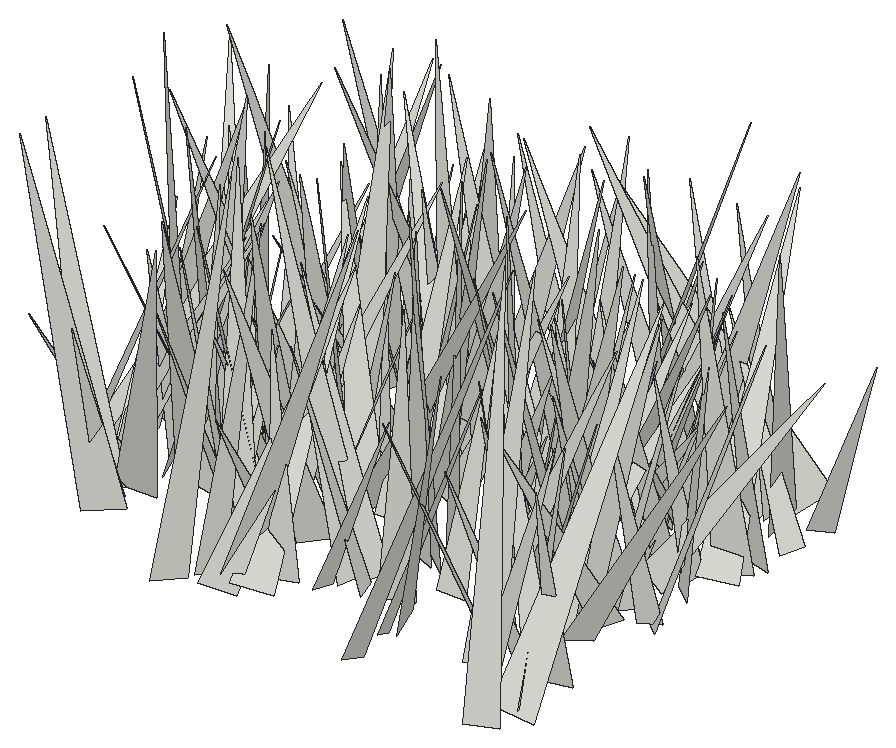
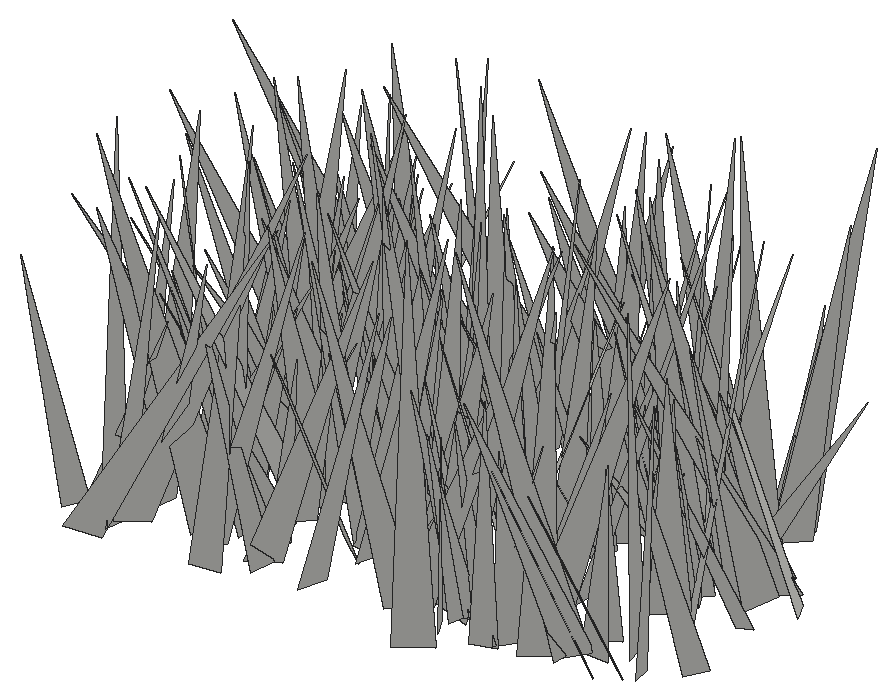
# SketchUp Ruby script. Lengths in inches.
U = 1.inch
M = Sketchup.active_model
def pt(a) = Geom::Point3d.new(a.map { |v| v * U })
def face(e, loops, mat)
  f = e.add_face(loops[0].map { |a| pt(a) })
  loops[1..].each { |l| e.add_face(l.map { |a| pt(a) }).erase! }
  f.material = f.back_material = mat if mat
  f
end
# faces: each face lists its corners as indices into pts; further lists are holes
def faces(e, pts, list, mat = nil) = list.each { |f| face(e, (f[0].is_a?(Array) ? f : [f]).map { |l| l.map { |i| pts[i] } }, mat) }
# xy, xz, yz: faces in a plane at the given z, y or x. An outline is a flat list of corners, or four numbers for a rectangle; further outlines are holes
def ring(l) = l.size == 4 ? [[l[0], l[1]], [l[2], l[1]], [l[2], l[3]], [l[0], l[3]]] : l.each_slice(2).to_a
def flat(e, list, mat, &to3) = list.each { |f| face(e, (f[0].is_a?(Array) ? f : [f]).map { |l| ring(l).map { |u, v| to3.(u, v) } }, mat) }
def xy(e, z, list, mat = nil) = flat(e, list, mat) { |x, y| [x, y, z] }
def xz(e, y, list, mat = nil) = flat(e, list, mat) { |x, z| [x, y, z] }
def yz(e, x, list, mat = nil) = flat(e, list, mat) { |y, z| [x, y, z] }
def lines(e, pts, list) = list.each { |a, b| e.add_line(pt(pts[a]), pt(pts[b])) }
# prism: a flat outline (further loops are holes) pulled along v
def prism(e, loops, v, mat = nil)
  f = face(e, loops, mat); d = Geom::Vector3d.new(v.map { |x| x * U })
  f.pushpull(f.normal.samedirection?(d) ? d.length : -d.length)
end
def box(e, o, s, mat = nil) = prism(e, [[o, [o[0] + s[0], o[1], o[2]], [o[0] + s[0], o[1] + s[1], o[2]], [o[0], o[1] + s[1], o[2]]]], [0, 0, s[2]], mat)
def at(x, y, z, deg = 0) = Geom::Transformation.translation(pt([x, y, z])) * Geom::Transformation.rotation(ORIGIN, Z_AXIS, deg.degrees)
def axes(o, x, y, z) = Geom::Transformation.new([*x, 0, *y, 0, *z, 0, *pt(o).to_a, 1])
def part(name) = M.definitions.add(name)
# library, detail: a bought-in or finely detailed component or shape, given as its bounding box
def library(name, o, s) = part(name).tap { |d| box(d.entities, o, s) }
def detail(e, o, s) = box(e.add_group.entities, o, s)
def put(e, d, t, mat = nil) = e.add_instance(d, t).tap { |i| i.material = mat if mat }
def group(e, t, mat = nil) = e.add_group.tap { |g| g.transformation = t; g.material = mat if mat }.entities
root = M.entities
c1 = part("fur_instance\#9")
p = [[0.8125,0,1.79],[0.67,-0.02,1.48],[0,-0.11,0],[0,0.11,0]]
faces(c1.entities,p,[[0,1,2,3]])
put(root,c1,axes([156.88,270.8125,-27.1],[4.55494,-1.38322,1.77977],[-1.90749,-4.50337,1.38185],[-1.20098,1.9065,4.55536]))
put(root,c1,axes([138.06,273.06,-27.1],[2.50523,-6.92108,2.84903],[-7.08461,-3.16179,-1.45116],[-2.41383,2.09672,7.21607]))
put(root,c1,axes([158.23,269.17,-27.1],[0.30584,8.28043,0.48557],[7.987,-0.4251,2.21855],[-2.2381,-0.38549,7.98355]))
put(root,c1,axes([151.5,273.3,-27.1],[6.22131,1.299,1.34326],[1.60809,-6.10017,-1.54868],[-0.95174,-1.81575,6.1639]))
put(root,c1,axes([158.52,273.24,-27.1],[1.07632,-4.38935,0.89904],[-4.4763,-1.09335,0.02097],[-0.19334,0.87825,4.51934]))
put(root,c1,axes([143.01,270.55,-27.1],[-6.71814,2.72987,2.53139],[2.23652,7.13443,-1.75826],[2.97626,0.8008,7.03521]))
put(root,c1,axes([155.51,273.35,-27.1],[-3.79986,-3.34827,0.10157],[-3.34083,3.7767,-0.4853],[-0.24505,0.43103,5.04126]))
put(root,c1,axes([137.81,273.82,-27.1],[2.72704,-3.27265,0.76108],[-3.17295,-2.83078,-0.80329],[-1.10537,0.05182,4.1835]))
put(root,c1,axes([138.07,274.83,-27.1],[2.36593,-6.95857,0.28973],[-6.83072,-2.25873,1.53056],[1.359,0.76137,7.18865]))
put(root,c1,axes([156.9,273.36,-27.1],[-0.5806,-4.0301,0.94816],[-3.96701,0.26756,-1.29192],[-1.18471,1.07913,3.86131]))
put(root,c1,axes([158.72,271.08,-27.1],[-4.5247,0.14497,1.56827],[-0.47946,4.4174,-1.79167],[1.5002,1.84904,4.15738]))
put(root,c1,axes([146.21,273.05,-27.1],[-1.45922,4.42701,2.15741],[4.90506,1.50733,0.22462],[0.43952,-2.12407,4.65589]))
put(root,c1,axes([144.89,271.98,-27.1],[7.47756,-1.51643,1.55812],[-1.8154,-7.42558,1.48539],[-1.19651,1.78955,7.48379]))
put(root,c1,axes([144.78,271.08,-27.1],[-3.66435,5.27166,1.90181],[4.6134,4.12758,-2.55233],[3.18179,0.08644,5.89097]))
put(root,c1,axes([151.63,270.18,-27.1],[7.3603,1.92647,1.4977],[1.22652,-7.03518,3.02165],[-2.10951,2.63124,6.98247]))
put(root,c1,axes([144.33,275.14,-27.1],[1.81992,-3.21241,0.00061],[-3.09433,-1.75321,-0.99152],[-0.86298,-0.48823,3.55649]))
put(root,c1,axes([143.84,271.83,-27.1],[-6.0255,1.4926,2.28597],[0.94971,6.33899,-1.63567],[2.5596,1.16168,5.98825]))
put(root,c1,axes([147.59,273.53,-27.1],[4.04534,-0.8517,0.30361],[-0.87788,-4.03293,0.38361],[-0.21657,0.43867,4.11619]))
put(root,c1,axes([158.59,270.49,-27.1],[-1.16046,8.00046,0.20395],[7.87345,1.17823,-1.41992],[1.43448,0.00519,7.95851]))
put(root,c1,axes([148.91,274.3125,-27.1],[-4.66141,-1.64687,0.68606],[-1.65466,4.70851,0.06011],[0.66704,0.1713,4.94341]))
put(root,c1,axes([145.32,276.02,-27.1],[2.99002,-5.93259,1.12286],[-5.76165,-3.17812,-1.449],[-1.8055,0.31717,6.48354]))
put(root,c1,axes([141.33,276.06,-27.1],[-4.0085,-3.44331,0.94309],[-3.06456,4.04605,1.74695],[1.83147,-0.76613,4.98725]))
put(root,c1,axes([150.23,274.4,-27.1],[2.8988,-5.16102,2.16058],[-5.5292,-3.01461,0.21733],[-0.85564,1.9958,5.91539]))
put(root,c1,axes([144.27,273.01,-27.1],[-5.43034,-1.89464,0.64767],[-1.9986,5.01546,-2.08529],[-0.12137,2.18018,5.36002]))
put(root,c1,axes([137.33,274.07,-27.1],[-5.93712,3.87569,1.72238],[4.1151,5.9813,0.72589],[1.02637,-1.56207,7.0529]))
put(root,c1,axes([151.37,272.24,-27.1],[4.47299,1.54799,0.88013],[1.09405,-4.26651,1.94385],[-1.40498,1.60599,4.31572]))
put(root,c1,axes([138.91,277.35,-27.1],[6.44625,-4.17663,0.34492],[-3.99481,-6.31514,-1.81045],[-1.26676,-1.33867,7.46462]))
put(root,c1,axes([137.73,275.46,-27.1],[-0.38653,-3.78857,0.47263],[-3.40937,0.1287,-1.7566],[-1.71837,0.59684,3.37891]))
put(root,c1,axes([155.375,272.83,-27.1],[-6.19625,3.45387,1.64148],[3.0912,6.3638,-1.72156],[2.25127,0.76815,6.88178]))
put(root,c1,axes([155.24,274.8125,-27.1],[-4.18009,-2.38384,1.39005],[-2.61185,4.23208,-0.59649],[0.8906,1.22265,4.77494]))
put(root,c1,axes([143.08,274.33,-27.1],[-2.11891,6.73628,2.3501],[7.12334,2.13432,0.30482],[0.39806,-2.33612,7.05509]))
put(root,c1,axes([143.9,275.12,-27.1],[-3.99562,-4.42007,1.47298],[-4.65768,3.83659,-1.12173],[0.11293,1.84803,5.85182]))
put(root,c1,axes([142.59,274.4,-27.1],[-0.05946,3.80591,1.08242],[3.88392,0.26301,-0.71143],[0.75616,-1.05166,3.7393]))
put(root,c1,axes([145.18,273.13,-27.1],[5.43487,-1.88004,3.06705],[-2.9758,-5.47185,1.91904],[-2.02138,3.00059,5.42123]))
put(root,c1,axes([148.13,274.78,-27.1],[-8.02945,1.44749,0.94959],[1.4539,8.08421,-0.0293],[0.93976,-0.13944,8.15883]))
put(root,c1,axes([154.01,276.96,-27.1],[0.47232,-5.02453,0.37853],[-5.03579,-0.45765,0.20889],[0.17316,0.39615,5.04235]))
put(root,c1,axes([156.79,274.1875,-27.1],[-1.63602,4.97918,0.62205],[4.87533,1.42244,1.43652],[-1.18757,-1.0199,5.04036]))
put(root,c1,axes([157.19,277.71,-27.1],[2.87484,-4.36178,0.57915],[-3.91954,-2.85297,-2.03053],[-1.99945,-0.67874,4.81319]))
put(root,c1,axes([145.75,271.82,-27.1],[-4.59589,5.78444,0.11594],[5.4804,4.40003,-2.28044],[1.8543,1.33244,7.02721]))
put(root,c1,axes([143.55,276.78,-27.1],[-0.33962,-4.53633,0.58104],[-4.49375,0.22275,-0.88758],[-0.84975,0.63509,4.46159]))
put(root,c1,axes([142.36,278.12,-27.1],[6.58115,-3.41587,1.26301],[-3.10443,-6.62563,-1.74311],[-1.90417,-1.00387,7.20703]))
put(root,c1,axes([148.61,275.26,-27.1],[-5.80532,1.01557,0.17125],[1.00882,5.80466,-0.22508],[0.20737,0.19232,5.88918]))
put(root,c1,axes([138.62,278.8125,-27.1],[-3.25593,-5.45811,0.05054],[-5.36708,3.21208,1.12765],[0.99394,-0.53501,6.25464]))
put(root,c1,axes([149.46,277.47,-27.1],[-3.95013,-6.45103,2.53754],[-6.55598,4.42551,1.04517],[2.25256,1.56763,7.49179]))
put(root,c1,axes([153.51,275.75,-27.1],[2.52048,5.79703,1.2985],[5.75928,-2.03853,-2.07834],[1.45681,-1.97061,5.96983]))
put(root,c1,axes([135.79,275.93,-27.1],[4.10268,4.53992,0.30052],[4.35228,-3.79801,-2.04106],[1.3262,-1.58032,5.76861]))
put(root,c1,axes([142.4,276.375,-27.1],[-2.65775,-2.55388,1.91088],[-2.80676,3.05414,0.17806],[1.51521,1.17784,3.68161]))
put(root,c1,axes([148.78,277.39,-27.1],[-1.6159,-6.90986,2.38073],[-7.13771,2.01606,1.00679],[1.57067,2.05292,7.0245]))
put(root,c1,axes([137.93,277.77,-27.1],[3.7662,-3.06911,1.25827],[-2.92554,-3.97067,-0.92842],[-1.56328,0.03677,4.76883]))
put(root,c1,axes([151.5,275.9,-27.1],[-0.63443,5.02312,1.44392],[5.17666,0.80438,-0.52377],[0.72032,-1.3566,5.03586]))
put(root,c1,axes([157.02,276.14,-27.1],[5.8068,-2.41673,0.19711],[-2.36119,-5.5195,1.88633],[0.55156,1.81463,6.0001]))
put(root,c1,axes([136.15,276.54,-27.1],[3.52755,5.08967,0.59914],[4.90233,-3.13928,-2.19532],[1.49362,-1.71683,5.79042]))
put(root,c1,axes([139.86,276.4,-27.1],[1.56528,5.39191,1.82425],[5.61252,-1.77733,0.43748],[-0.9488,-1.61836,5.59744]))
put(root,c1,axes([155.9,277.65,-27.1],[-2.90009,-5.61636,1.60668],[-5.82709,2.65472,-1.23809],[-0.41218,1.98605,6.19848]))
put(root,c1,axes([153.88,278.1875,-27.1],[4.89387,1.35478,0.49174],[1.44124,-4.60961,-1.64362],[-0.00784,-1.71558,4.80457]))
put(root,c1,axes([146.14,277.15,-27.1],[3.85266,4.81198,3.39076],[5.17881,-4.69725,0.78179],[-2.79863,-2.06788,6.11449]))
put(root,c1,axes([155.28,279.84,-27.1],[3.26606,-6.16963,0.62937],[-6.14796,-3.31446,-0.58694],[-0.81426,0.27855,6.95607]))
put(root,c1,axes([138.24,279.3,-27.1],[-6.05203,-3.65216,2.90127],[-3.20675,6.70926,1.75646],[3.38709,-0.1736,6.84691]))
put(root,c1,axes([142.83,279.54,-27.1],[-3.8372,-2.33717,0.79383],[-2.01321,3.81242,1.493],[1.42812,-0.90538,4.23762]))
put(root,c1,axes([153.32,277.49,-27.1],[-6.66859,-2.01923,2.71074],[-2.32845,7.09045,-0.44648],[2.45024,1.24248,6.95328]))
put(root,c1,axes([158.25,278.68,-27.1],[1.30026,-4.12004,1.09762],[-4.18224,-1.45572,-0.50983],[-0.82967,0.8811,4.29016]))
put(root,c1,axes([136.82,275.79,-27.1],[-2.17484,4.53028,0.06229],[4.50087,2.16823,-0.54601],[0.51907,0.1805,4.99552]))
put(root,c1,axes([133.94,277.78,-27.1],[5.98281,3.47845,0.55141],[3.51313,-5.81778,-1.41742],[0.2481,-1.50052,6.77381]))
put(root,c1,axes([137.92,276.9,-27.1],[6.78168,2.91502,1.19431],[2.8839,-6.88568,0.43057],[-1.26762,-0.07012,7.36906]))
put(root,c1,axes([155.07,279.76,-27.1],[1.17594,-4.92519,0.34785],[-4.93492,-1.18388,-0.07952],[-0.1583,0.31979,5.06301]))
put(root,c1,axes([139.65,277.89,-27.1],[3.10895,3.01642,1.49943],[3.22004,-3.26039,-0.11754],[-0.98914,-1.13301,4.33019]))
put(root,c1,axes([151.19,278.72,-27.1],[2.68666,-2.71893,0.01615],[-2.65256,-2.616,0.85524],[0.59729,0.61233,3.72549]))
put(root,c1,axes([153.03,278.02,-27.1],[3.30994,1.56111,0.94089],[1.62723,-3.40964,-0.0672],[-0.82125,-0.46405,3.659]))
put(root,c1,axes([140.05,277.67,-27.1],[3.54809,3.00738,1.07129],[3.07779,-3.64774,0.04651],[-0.84804,-0.65624,4.65093]))
put(root,c1,axes([142.13,278.7,-27.1],[2.86459,-3.18276,1.27512],[-3.34476,-2.95943,0.1272],[-0.754,1.03614,4.28015]))
put(root,c1,axes([153.55,278.46,-27.1],[-3.32572,-4.76152,1.64129],[-5.0351,3.09772,-1.21581],[-0.11678,2.03921,5.67929]))
put(root,c1,axes([141.63,276.95,-27.1],[-0.67642,4.08917,0.12939],[3.98053,0.62749,0.97839],[-0.94522,-0.2838,4.0276]))
put(root,c1,axes([137.56,278.46,-27.1],[3.65064,-1.60023,0.53489],[-1.66152,-3.63138,0.47591],[-0.29361,0.65299,3.95745]))
put(root,c1,axes([142.9,277.91,-27.1],[0.16923,4.07191,1.2027],[4.12697,0.12503,-1.00402],[0.99752,-1.2081,3.94982]))
put(root,c1,axes([155.28,278.67,-27.1],[0.56131,-6.10589,2.64479],[-6.41112,0.21442,1.85565],[1.78167,2.69518,5.8441]))
put(root,c1,axes([138.05,277.61,-27.1],[3.6249,6.4726,3.15784],[6.5149,-4.45394,1.65071],[-3.06961,-1.8095,7.23254]))
put(root,c1,axes([156,276.26,-27.1],[0.77683,6.56918,0.32302],[6.56801,-0.79193,0.30978],[-0.34589,-0.28401,6.60769]))
put(root,c1,axes([157.04,278.98,-27.1],[-1.11932,5.12608,2.18052],[5.30702,0.30525,2.00664],[-1.6932,-2.43194,4.84799]))
put(root,c1,axes([135.375,278.34,-27.1],[6.77248,-2.83159,1.61361],[-3.13932,-6.6674,1.47599],[-0.87537,2.00399,7.19067]))
put(root,c1,axes([137.61,279.39,-27.1],[5.01911,-5.50348,2.14134],[-5.83765,-5.04831,0.7082],[-0.89193,2.07156,7.41473]))
put(root,c1,axes([140.43,281.86,-27.1],[-7.65526,-2.65251,1.50577],[-2.23878,7.64939,2.09305],[2.07148,-1.53532,7.82675]))
put(root,c1,axes([136.4,280.93,-27.1],[-5.36571,-5.00333,1.81378],[-4.95811,5.63559,0.87824],[1.93398,0.5664,7.28374]))
put(root,c1,axes([145.28,278.87,-27.1],[7.55011,-1.58138,0.22082],[-1.59514,-7.42262,1.38345],[0.0711,1.39915,7.58887]))
put(root,c1,axes([135.15,277.13,-27.1],[0.81957,8.13408,0.73803],[7.68253,-0.51597,-2.84467],[2.77248,-0.97476,7.66439]))
put(root,c1,axes([152.63,280.28,-27.1],[7.05562,-2.47543,1.6862],[-2.53392,-7.23407,-0.01726],[-1.59697,0.54154,7.47725]))
put(root,c1,axes([152.8,280.89,-27.1],[2.44609,-6.94499,1.47158],[-6.99231,-2.08787,1.76924],[1.22722,1.94671,7.14745]))
put(root,c1,axes([152.75,277.01,-27.1],[1.27817,7.72916,0.81529],[7.27012,-1.48113,2.64386],[-2.74773,-0.32349,7.37453]))
put(root,c1,axes([149.71,278.17,-27.1],[-6.21182,-1.68937,2.27799],[-2.42044,6.01654,-2.13837],[1.47806,2.75267,6.07191]))
put(root,c1,axes([135.25,279.7,-27.1],[2.3418,4.95634,1.60959],[5.19702,-2.35112,-0.32146],[-0.38351,-1.59595,5.4723]))
put(root,c1,axes([141.39,282.09,-27.1],[5.68928,-3.36377,1.44998],[-3.11585,-5.85243,-1.35122],[-1.92583,-0.46842,6.46971]))
put(root,c1,axes([147.45,278.09,-27.1],[5.41894,2.39891,1.8987],[1.67708,-5.5593,2.23748],[-2.55876,1.4367,5.48756]))
put(root,c1,axes([154.06,278.99,-27.1],[2.83544,5.2975,1.05869],[5.3487,-2.92083,0.29014],[-0.75876,-0.79328,6.00159]))
put(root,c1,axes([138.41,278.5,-27.1],[3.83996,1.68055,0.1423],[1.49178,-3.54944,1.66307],[-0.78682,1.47206,3.84756]))
put(root,c1,axes([146.5625,278.84,-27.1],[-1.26821,6.79621,1.34265],[6.86908,1.41065,-0.65215],[0.89826,-1.19212,6.8827]))
put(root,c1,axes([156.75,278.38,-27.1],[2.63197,4.07891,0.20518],[3.86496,-2.5665,1.44292],[-1.31973,0.61842,4.63495]))
put(root,c1,axes([138.45,279.76,-27.1],[-1.05429,4.67357,0.99792],[4.75005,0.91265,0.74413],[-0.52453,-1.12891,4.73287]))
put(root,c1,axes([137.33,279.15,-27.1],[3.31155,2.43431,1.59522],[1.82743,-3.61986,1.73033],[-2.2652,0.63849,3.72802]))
put(root,c1,axes([134.72,279.9375,-27.1],[1.36791,4.73736,0.76135],[4.55305,-1.0318,-1.76027],[1.51392,-1.17738,4.60599]))
put(root,c1,axes([152.19,280.03,-27.1],[3.72107,-3.56028,1.90501],[-4.03778,-3.30047,1.71878],[-0.03061,2.5656,4.85467]))
put(root,c1,axes([153.92,280.49,-27.1],[-4.56501,-1.69942,1.47091],[-1.97129,4.62695,-0.77219],[1.07964,1.26263,4.80947]))
put(root,c1,axes([149.29,281.62,-27.1],[1.54528,-3.8993,0.59524],[-3.77652,-1.27799,1.43226],[1.13873,1.05307,3.94222]))
put(root,c1,axes([158.62,278.38,-27.1],[3.88995,3.95886,0.07672],[3.75671,-3.72392,1.68217],[-1.25122,1.12695,5.2891]))
put(root,c1,axes([146.85,281.06,-27.1],[7.17764,0.6661,2.04171],[0.73913,-7.45363,-0.1667],[-2.01642,-0.36113,7.20655]))
put(root,c1,axes([147.49,280.95,-27.1],[1.43912,5.66343,2.07225],[5.60003,-0.46439,-2.61988],[2.23794,-2.47985,5.22319]))
put(root,c1,axes([155.02,282.1,-27.1],[-0.84306,-4.44176,0.86686],[-4.52258,0.85891,0.00263],[0.16427,0.85115,4.52106]))
put(root,c1,axes([154.27,278.98,-27.1],[-0.54715,4.89077,0.10405],[4.53126,0.54616,-1.84371],[1.84341,0.10915,4.56287]))
put(root,c1,axes([156.3125,282.11,-27.1],[0.08099,-5.17118,1.20761],[-5.27072,-0.22549,-0.61212],[-0.64729,1.18913,5.13546]))
put(root,c1,axes([143.2,280.11,-27.1],[3.15167,2.15202,0.19961],[2.1362,-3.1554,0.29004],[-0.32814,0.12762,3.80527]))
put(root,c1,axes([148.56,283.95,-27.1],[-2.04467,-7.63412,0.65301],[-7.56547,2.11851,1.07815],[1.21235,0.345,7.82931]))
put(root,c1,axes([152.45,282.29,-27.1],[-1.50167,-7.67594,2.08534],[-7.92089,1.24921,-1.10571],[-0.72669,2.24569,7.7429]))
put(root,c1,axes([142.38,284.2,-27.1],[-4.33714,-4.09832,0.0827],[-3.81397,4.0787,2.10515],[1.50223,-1.4771,5.58349]))
put(root,c1,axes([143.84,280.56,-27.1],[-4.18107,4.06515,1.12452],[4.17237,4.21812,0.26475],[0.61747,-0.97641,5.82552]))
put(root,c1,axes([157.47,282.13,-27.1],[-4.17455,0.44699,1.70239],[0.80041,4.38471,0.81146],[1.56757,-1.04848,4.11925]))
put(root,c1,axes([154.5,281.54,-27.1],[-3.00148,-2.27694,0.1564],[-2.20162,2.82047,-1.1898],[-0.60148,1.03841,3.57459]))
put(root,c1,axes([153.21,281.91,-27.1],[6.75875,-1.16964,0.00047],[-1.16859,-6.75255,0.29358],[0.0496,0.28936,6.85293]))
put(root,c1,axes([142.48,281.96,-27.1],[2.08402,3.38406,1.47593],[3.68931,-1.84524,-0.97848],[0.13865,-1.76538,3.85196]))
put(root,c1,axes([151.42,281.67,-27.1],[-2.68831,3.38264,1.06218],[3.54497,2.54168,0.8778],[-0.06058,-1.37662,4.23069]))
put(root,c1,axes([141.0625,279.95,-27.1],[2.76171,5.55128,0.00194],[5.48471,-2.72826,-0.95829],[0.85713,-0.42855,6.1258]))
put(root,c1,axes([157.875,281.02,-27.1],[3.73887,4.62596,1.90486],[4.75099,-4.02818,0.45718],[-1.5672,-1.17533,5.9304]))
put(root,c1,axes([138.22,280.77,-27.1],[-1.29816,5.29172,0.79515],[5.27739,1.13069,1.0911],[-0.88529,-1.01932,5.33826]))
put(root,c1,axes([146.02,283.03,-27.1],[-0.11111,-7.60969,2.49454],[-7.52897,0.94928,2.56048],[2.72852,2.30953,7.16685]))
put(root,c1,axes([156.36,281.14,-27.1],[1.31269,5.55847,0.82299],[4.82858,-0.68361,-3.08457],[2.8738,-1.39037,4.80678]))
put(root,c1,axes([153.85,280.31,-27.1],[-1.09311,5.26549,0.63584],[5.05113,1.23151,-1.51458],[1.61731,-0.28736,5.16007]))
put(root,c1,axes([156.67,283.4,-27.1],[-1.81586,-4.37557,0.34615],[-4.20637,1.62778,-1.48984],[-1.25376,0.87607,4.49704]))
put(root,c1,axes([158.36,283.28,-27.1],[-2.64442,5.36733,3.49605],[6.32318,2.79183,0.49668],[1.02376,-3.3795,5.96276]))
put(root,c1,axes([142.53,281.59,-27.1],[-5.26533,5.42334,2.66225],[5.51698,5.75546,-0.81326],[2.46233,-1.29842,7.51498]))
put(root,c1,axes([151.46,281.49,-27.1],[-5.91196,3.62871,1.99788],[3.48429,6.23911,-1.02156],[2.24027,-0.12769,6.86114]))
put(root,c1,axes([137.45,280.78,-27.1],[-4.42637,5.44798,0.10976],[5.44745,4.42761,-0.08267],[0.13338,-0.03304,7.019]))
put(root,c1,axes([151.6875,283.5625,-27.1],[-3.71371,1.13934,1.58672],[1.47505,3.87017,0.67337],[1.28063,-1.15373,3.82574]))
put(root,c1,axes([149.36,282.98,-27.1],[7.16515,0.1083,1.44204],[0.09788,-7.3087,0.06254],[-1.44279,0.042,7.1657]))
put(root,c1,axes([155.14,282.3125,-27.1],[-1.55107,4.41542,0.77186],[4.34501,1.28043,1.40671],[-1.10114,-1.16708,4.46351]))
put(root,c1,axes([134.03,283.55,-27.1],[2.085,-4.49657,0.98747],[-4.39792,-1.62495,1.88661],[1.36107,1.63764,4.58334]))
put(root,c1,axes([141.14,283.3,-27.1],[-1.13244,4.66111,1.93868],[4.91983,0.57378,1.4943],[-1.13125,-2.17064,4.55801]))
put(root,c1,axes([158.625,284.28,-27.1],[-1.20745,-5.31811,1.49773],[-5.50418,1.29079,0.14593],[0.47907,1.42653,5.45151]))
put(root,c1,axes([139.22,286.05,-27.1],[6.38115,-3.67921,0.2036],[-3.55943,-6.25987,-1.56256],[-0.95316,-1.25481,7.1982]))
put(root,c1,axes([136.625,283.61,-27.1],[-5.78196,-1.74059,3.08913],[-1.82129,6.52793,0.26926],[3.04225,0.59997,6.03227]))
put(root,c1,axes([146.49,282.5,-27.1],[0.66704,7.88186,2.68055],[8.14998,-1.16705,1.40349],[-1.69907,-2.50365,7.78452]))
put(root,c1,axes([155.61,281.47,-27.1],[3.29969,3.36632,0.10349],[3.25213,-3.22241,1.12716],[-0.87548,0.71745,4.57707]))
put(root,c1,axes([142.9375,282.45,-27.1],[1.28068,6.67783,2.12971],[6.86225,-1.63556,1.00185],[-1.42781,-1.87102,6.72532]))
put(root,c1,axes([146.75,282.2,-27.1],[-4.59485,5.55244,0.46156],[5.5505,4.50971,1.00485],[-0.48434,-0.99407,7.1367]))
put(root,c1,axes([140.03,284.67,-27.1],[-0.48012,-7.554,2.16495],[-7.6037,-0.10085,-2.03814],[-1.98335,2.21526,7.28968]))
put(root,c1,axes([146.01,285.4,-27.1],[4.30794,-3.29071,0.86204],[-3.07513,-4.36194,-1.28347],[-1.45447,-0.52435,5.26686]))
put(root,c1,axes([144,281.72,-27.1],[3.8094,4.08661,1.06154],[3.80016,-3.94157,1.53675],[-1.84012,0.32005,5.37125]))
put(root,c1,axes([137.83,283.6,-27.1],[1.56835,-2.82264,1.69633],[-3.20586,-1.73838,0.07137],[-0.75322,1.52161,3.2283]))
put(root,c1,axes([155.58,282.45,-27.1],[3.89268,2.82638,0.90518],[2.67493,-3.98806,0.94914],[-1.28551,0.26015,4.71599]))
put(root,c1,axes([152.82,283.86,-27.1],[2.65844,-2.5721,0.0216],[-2.2994,-2.3625,1.67773],[1.15278,1.21916,3.2967]))
put(root,c1,axes([144.21,285.18,-27.1],[4.56733,-2.95407,1.62637],[-2.80415,-4.84794,-0.93072],[-1.87305,0.05455,5.35918]))
put(root,c1,axes([135.47,284.86,-27.1],[-4.30625,-1.78107,2.16646],[-1.55574,4.81995,0.87021],[2.33354,-0.07334,4.57807]))
put(root,c1,axes([148.45,283.22,-27.1],[-1.13275,3.97734,1.11963],[3.98013,1.3621,-0.81189],[1.10966,-0.82546,4.05502]))
put(root,c1,axes([152.58,281.61,-27.1],[-6.84761,2.51212,1.52779],[1.98246,6.80446,-2.30302],[2.17135,1.70976,6.92074]))
put(root,c1,axes([140.39,285.84,-27.1],[7.09602,-3.54407,1.49132],[-3.45875,-7.25092,-0.77408],[-1.67974,-0.04148,7.89397]))
put(root,c1,axes([148.15,284.06,-27.1],[-7.39383,1.79038,1.19471],[1.82356,7.48136,0.07416],[1.14343,-0.35412,7.60715]))
put(root,c1,axes([142.66,285.18,-27.1],[4.32257,0.5968,0.21737],[0.63053,-4.21214,-0.97382],[-0.07654,-0.99484,4.25352]))
put(root,c1,axes([153.93,284.82,-27.1],[2.87262,5.81566,3.24646],[6.49078,-3.23727,0.05584],[-1.49368,-2.88298,6.48619]))
put(root,c1,axes([144.61,286.43,-27.1],[-1.86183,-7.54983,1.10161],[-7.50699,1.61006,-1.65309],[-1.3633,1.44488,7.59827]))
put(root,c1,axes([143.7,285.52,-27.1],[-0.98581,-7.65367,2.64082],[-7.9173,0.35473,-1.92744],[-1.69382,2.79641,7.47232]))
put(root,c1,axes([142,285.25,-27.1],[-3.00946,-2.45302,0.73779],[-2.54129,3.00205,-0.38468],[0.32167,0.76736,3.86344]))
put(root,c1,axes([151.49,285.28,-27.1],[1.53479,-3.08573,1.52348],[-3.30012,-1.79268,-0.30636],[-0.97569,1.2095,3.43271]))
put(root,c1,axes([138.42,285.18,-27.1],[7.76844,-0.71206,0.72464],[-0.74639,-7.79129,0.34557],[-0.68922,0.41169,7.79335]))
put(root,c1,axes([157.37,287.27,-27.1],[7.02659,-0.33713,1.59],[0.09653,-6.95626,-1.90152],[-1.62247,-1.87389,6.7728]))
put(root,c1,axes([141.45,286.15,-27.1],[1.4619,-3.63585,0.57448],[-3.60479,-1.28901,1.01518],[0.74496,0.89757,3.78497]))
put(root,c1,axes([152.41,284.83,-27.1],[3.65176,6.04586,1.11201],[6.02251,-3.25936,-2.05677],[1.23222,-1.98709,6.75703]))
put(root,c1,axes([152.82,285.41,-27.1],[5.19271,0.37939,0.34653],[0.38191,-5.20401,-0.02543],[-0.34375,-0.05067,5.20649]))
put(root,c1,axes([158.19,282.58,-27.1],[-3.4412,6.39637,0.09759],[6.32165,3.41718,-1.06042],[0.97968,0.41743,7.18546]))
put(root,c1,axes([152.48,282.82,-27.1],[7.12213,3.78972,1.00867],[3.4176,-7.02352,2.25704],[-1.92338,1.55314,7.74548]))
put(root,c1,axes([156.5,287.42,-27.1],[-7.92246,2.32052,1.49756],[2.68865,7.5204,2.57051],[0.63138,-2.90715,7.84491]))
put(root,c1,axes([152.32,288.47,-27.1],[-1.3783,-7.92591,0.91068],[-7.76861,1.54372,1.6777],[1.81604,0.58822,7.86798]))
put(root,c1,axes([137.57,284.89,-27.1],[-1.32199,4.73147,0.88748],[4.77716,1.17578,0.84759],[-0.59431,-1.0737,4.83901]))
put(root,c1,axes([150.99,286.82,-27.1],[-5.87282,3.13064,1.60123],[3.47052,5.66214,1.65846],[0.56601,-2.23474,6.44519]))
put(root,c1,axes([153.12,287.1,-27.1],[-6.41083,1.14128,1.69671],[1.48537,6.43646,1.28286],[1.40536,-1.59673,6.38401]))
put(root,c1,axes([136.06,285.3125,-27.1],[2.47782,3.1575,0.0552],[3.13992,-2.45577,-0.47176],[0.33732,-0.3344,3.98583]))
put(root,c1,axes([158.9375,285.9,-27.1],[-4.27711,1.68369,0.0136],[1.68167,4.26988,0.26227],[-0.08344,-0.24902,4.58909]))
put(root,c1,axes([145.12,286.34,-27.1],[-0.35143,6.05342,2.99786],[6.31844,1.35633,-1.99808],[2.38924,-2.69649,5.72495]))
put(root,c1,axes([153.92,285.9375,-27.1],[6.10397,-4.61293,1.81963],[-4.95361,-5.80478,1.9013],[-0.22786,2.62185,7.41098]))
put(root,c1,axes([141.15,286.7,-27.1],[1.68942,-4.24341,1.91691],[-4.60334,-1.82876,0.00876],[-0.70022,1.78447,4.56734]))
put(root,c1,axes([143.02,285.63,-27.1],[3.50267,-1.34823,2.1537],[-1.97697,-3.75014,0.86764],[-1.59615,1.68627,3.65152]))
put(root,c1,axes([143.03,288.29,-27.1],[3.4393,-6.56896,1.063],[-6.65437,-3.3911,0.57422],[0.02233,1.20797,7.39258]))
put(root,c1,axes([143.21,286.58,-27.1],[3.08289,1.97486,1.70839],[2.08981,-3.45082,0.21788],[-1.56569,-0.71742,3.6547]))
put(root,c1,axes([142.81,285.5,-27.1],[-1.16488,5.07104,1.08343],[5.11451,1.30667,-0.61696],[0.85504,-0.90739,5.16641]))
put(root,c1,axes([150.79,287.14,-27.1],[5.32067,-0.59583,0.38531],[-0.58759,-5.33383,-0.13414],[-0.39777,-0.09079,5.35224]))
put(root,c1,axes([149.07,284.23,-27.1],[2.7978,5.22834,0.27095],[4.99402,-2.75746,1.64099],[-1.57121,0.54549,5.69828]))
put(root,c1,axes([148.62,287.03,-27.1],[-6.00997,1.04438,1.22572],[1.13938,6.10462,0.38513],[1.13796,-0.59647,6.08787]))
put(root,c1,axes([156.42,285.89,-27.1],[-6.22467,1.67352,0.58559],[1.62437,6.23957,-0.56507],[0.71064,0.39649,6.42089]))
put(root,c1,axes([158.81,287.64,-27.1],[3.25053,-3.28963,0.28157],[-3.26975,-3.15258,0.91484],[0.45796,0.84053,4.53329]))
put(root,c1,axes([157.35,289.11,-27.1],[-6.27712,3.42033,1.55819],[3.73626,5.34865,3.31076],[-0.40863,-3.63622,6.33559]))
put(root,c1,axes([156.74,287.79,-27.1],[5.59524,-0.57904,3.08549],[-0.36766,-6.38318,-0.53118],[-3.11775,-0.28642,5.59999]))
put(root,c1,axes([137.09,285.8,-27.1],[2.95968,3.81178,0.17357],[3.80838,-2.96454,0.16477],[-0.23661,-0.0359,4.82309]))
put(root,c1,axes([138.15,285.2,-27.1],[-2.51338,5.74575,1.01303],[5.46798,2.70448,-1.77311],[2.03497,-0.17044,6.01555]))
